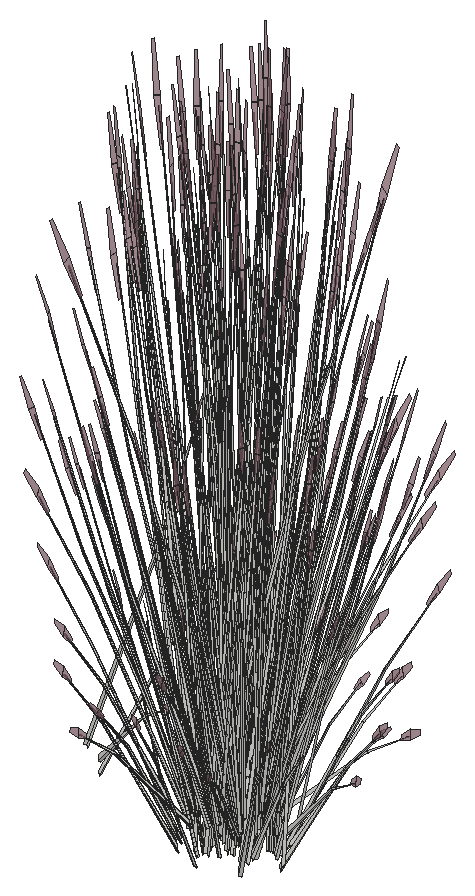
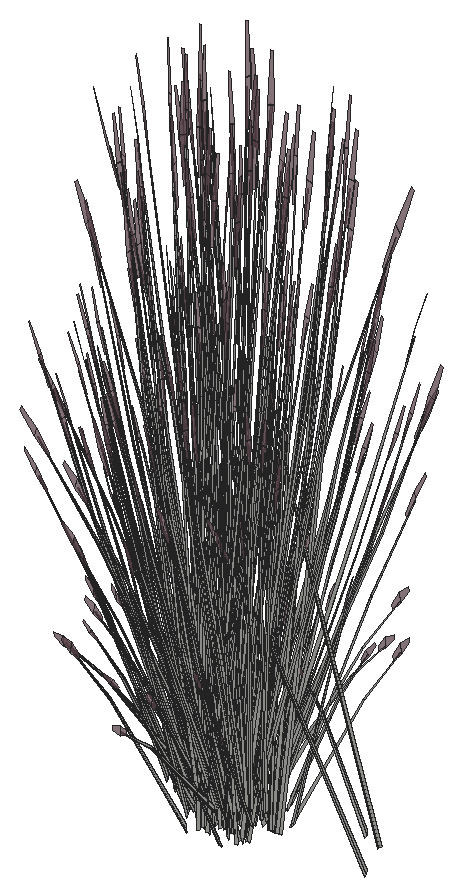
# SketchUp Ruby script. Lengths in inches.
U = 1.inch
M = Sketchup.active_model
def pt(a) = Geom::Point3d.new(a.map { |v| v * U })
def face(e, loops, mat)
  f = e.add_face(loops[0].map { |a| pt(a) })
  loops[1..].each { |l| e.add_face(l.map { |a| pt(a) }).erase! }
  f.material = f.back_material = mat if mat
  f
end
# faces: each face lists its corners as indices into pts; further lists are holes
def faces(e, pts, list, mat = nil) = list.each { |f| face(e, (f[0].is_a?(Array) ? f : [f]).map { |l| l.map { |i| pts[i] } }, mat) }
# xy, xz, yz: faces in a plane at the given z, y or x. An outline is a flat list of corners, or four numbers for a rectangle; further outlines are holes
def ring(l) = l.size == 4 ? [[l[0], l[1]], [l[2], l[1]], [l[2], l[3]], [l[0], l[3]]] : l.each_slice(2).to_a
def flat(e, list, mat, &to3) = list.each { |f| face(e, (f[0].is_a?(Array) ? f : [f]).map { |l| ring(l).map { |u, v| to3.(u, v) } }, mat) }
def xy(e, z, list, mat = nil) = flat(e, list, mat) { |x, y| [x, y, z] }
def xz(e, y, list, mat = nil) = flat(e, list, mat) { |x, z| [x, y, z] }
def yz(e, x, list, mat = nil) = flat(e, list, mat) { |y, z| [x, y, z] }
def lines(e, pts, list) = list.each { |a, b| e.add_line(pt(pts[a]), pt(pts[b])) }
# prism: a flat outline (further loops are holes) pulled along v
def prism(e, loops, v, mat = nil)
  f = face(e, loops, mat); d = Geom::Vector3d.new(v.map { |x| x * U })
  f.pushpull(f.normal.samedirection?(d) ? d.length : -d.length)
end
def box(e, o, s, mat = nil) = prism(e, [[o, [o[0] + s[0], o[1], o[2]], [o[0] + s[0], o[1] + s[1], o[2]], [o[0], o[1] + s[1], o[2]]]], [0, 0, s[2]], mat)
def at(x, y, z, deg = 0) = Geom::Transformation.translation(pt([x, y, z])) * Geom::Transformation.rotation(ORIGIN, Z_AXIS, deg.degrees)
def axes(o, x, y, z) = Geom::Transformation.new([*x, 0, *y, 0, *z, 0, *pt(o).to_a, 1])
def part(name) = M.definitions.add(name)
# library, detail: a bought-in or finely detailed component or shape, given as its bounding box
def library(name, o, s) = part(name).tap { |d| box(d.entities, o, s) }
def detail(e, o, s) = box(e.add_group.entities, o, s)
def put(e, d, t, mat = nil) = e.add_instance(d, t).tap { |i| i.material = mat if mat }
def group(e, t, mat = nil) = e.add_group.tap { |g| g.transformation = t; g.material = mat if mat }.entities
root = M.entities
M.materials.add("LightPink_Translucent").color = [144, 107, 117]
M.materials["LightPink_Translucent"].alpha = 0.75
c1 = part("blade")
p = [[2.15,0.21,22],[0,0.17,0],[0.09,0.45,0],[2.18,0.31,22],[2.29,0.31,22],[0.38,0.45,0],
  [2.48,0.24,33],[2.49,0.24,33],[2.48,0.22,33]]
faces(c1.entities,p,[[0,1,2,3],[4,5,2,3],[6,3,4,7],[8,0,3,6]])
c2 = part("seeds")
p = [[0.3,-0.1,1.38],[-0.01,-0.03,1.59],[-0.01,-0.03,0.03],[0.14,-0.07,-0.07],[0.29,-0.03,3],[0.15,0.01,3.11]]
faces(c2.entities,p,[[0,1,2,3],[1,0,4,5]],"LightPink_Translucent")
c3 = part("blade with seeds")
put(c3.entities,c1,at(0,0,0))
put(c3.entities,c2,axes([2.4,0.25,30.99],[1.5799,-0.05474,1.17369],[-0.12525,1.92788,0.29478],[-0.07173,-0.02425,1.56792]))
put(root,c3,axes([496.08,108.5625,4.17],[0.66765,-0.26986,-0.71045],[0.37208,0.55551,0.08574],[0.32259,-0.0631,1.00501]))
put(root,c3,axes([506.71,109.3125,3.875],[0.19519,0.55794,-0.51099],[-0.73919,0.0976,-0.3958],[-0.21183,0.14986,0.97773]))
put(root,c3,axes([506.92,106.35,3.92],[0.03826,-0.46465,0.0643],[0.57772,0.01274,0.50621],[-0.2213,-0.04862,0.77189]))
put(root,c3,axes([505.5625,110.32,3.91],[-0.01889,0.12092,1.74944],[0.53598,0.42065,-0.27667],[-0.14032,0.19892,0.14031]))
put(root,c3,axes([508.56,108.91,1.25],[-0.79037,-0.10018,-0.62353],[0.16679,-0.61794,-0.16365],[-0.23587,-0.07488,1.37633]))
put(root,c3,axes([508.7,105.54,4.62],[-0.50709,0.58578,-0.13619],[-0.73436,-0.33748,-0.75594],[-0.25527,-0.1655,1.14864]))
put(root,c3,axes([498.33,107.97,3.91],[0.10543,-0.09307,1.74944],[-0.13495,-0.57092,-0.27667],[0.26455,-0.10825,0.14031]))
put(root,c3,axes([507.31,106.69,4.24],[0.43232,0.38257,0.35414],[-0.49364,0.36215,-0.4572],[-0.25081,-0.0551,0.87481]))
put(root,c3,axes([508.48,106.02,4.17],[-0.64788,-0.29534,-0.71045],[0.46044,-0.51755,0.08574],[-0.23473,-0.17635,1.00501]))
put(root,c3,axes([508.18,106.03,3.875],[-0.74975,0.14525,-0.51099],[-0.13115,-0.55007,-0.3958],[-0.20138,-0.15763,0.97773]))
put(root,c3,axes([497.11,109.38,1.78],[-0.18299,-0.15028,1.43002],[0.23809,-0.49714,-0.30754],[0.37023,0.06735,0.61141]))
put(root,c3,axes([507.52,110.08,1.21],[-0.7111,-0.30552,-0.49651],[0.42504,-0.54784,0],[-0.16196,-0.06958,1.57504]))
put(root,c3,axes([507.21,105.53,0.6875],[-0.0736,0.08049,1.76342],[-0.74378,0.17355,-0.26939],[-0.17968,-0.15788,0.30037]))
put(root,c3,axes([506.37,108.91,4.23],[0.70283,0.33692,-0.1216],[-0.40491,0.48793,-0.67495],[-0.19857,0.16961,1.02557]))
put(root,c3,axes([507.95,110.45,1.57],[-0.47504,0.61229,0],[-0.79476,-0.34146,-0.51607],[-0.18101,-0.07777,1.63711]))
put(root,c3,axes([505.21,110.38,4.84],[0.67048,0.16311,-0.06488],[-0.20625,0.50201,-0.29416],[-0.10966,0.07622,0.97024]))
put(root,c3,axes([506.71,108.96,4.24],[0.66138,-0.08733,0.35414],[0.17464,0.49921,-0.4572],[-0.18953,0.13408,0.87481]))
put(root,c3,axes([507.09,111.34,1.78],[0.23977,-0.09639,1.43002],[0.59198,0.29065,-0.30754],[-0.1762,0.25149,0.61141]))
put(root,c3,axes([506.75,105.84,1.32],[-0.21918,0.49894,-0.03893],[-0.6746,-0.15348,-0.17649],[-0.10242,-0.08161,0.58215]))
put(root,c3,axes([508.5,104.15,3.9],[-0.01417,0.07324,1.77383],[-0.6991,0.2658,-0.16761],[-0.20573,-0.13587,0.31391]))
put(root,c3,axes([507.75,105.21,1.78],[-0.04601,0.19989,1.43002],[-0.67263,0.16733,-0.30754],[-0.15723,-0.25836,0.61141]))
put(root,c3,axes([507.97,105.73,3.07],[0.17368,0.19618,1.71376],[-0.80256,0.16516,0.13857],[-0.18139,-0.30799,0.73262]))
put(root,c3,axes([509.45,109,1.86],[-0.76714,0.40567,-0.29095],[-0.51013,-0.57321,-0.50002],[-0.18927,-0.05821,1.59708]))
put(root,c3,axes([507.33,110.29,3.93],[-0.54105,-0.41691,0.48003],[0.57458,-0.35956,0.3958],[-0.0998,0.1956,0.9933]))
put(root,c3,axes([508.26,105.63,3.72],[-0.11735,-0.49217,-0.35414],[0.67083,-0.12996,0.4572],[-0.18018,-0.14104,0.87481]))
put(root,c3,axes([506.38,108.12,1.57],[-0.95008,0,0],[0,-0.68292,-0.51607],[0,-0.15554,1.63711]))
put(root,c3,axes([507.72,109.85,1.22],[-0.17848,-0.53243,-0.30978],[0.70886,-0.15119,0.30978],[-0.1429,-0.0614,1.38974]))
put(root,c3,axes([507.14,110.25,3.92],[-0.62439,-0.02847,0.0643],[0.01712,-0.42991,0.50621],[-0.06534,0.16468,0.77189]))
put(root,c3,axes([507.33,110.41,3.72],[-0.5141,0.32171,-0.35414],[-0.48666,-0.36734,0.4572],[-0.07405,0.18664,0.87481]))
put(root,c3,axes([509.96,109.45,1.25],[-0.51177,0.45928,-0.62353],[-0.63575,-0.41646,-0.16365],[-0.20507,0.11457,1.37633]))
put(root,c3,axes([508.65,106.03,4.24],[0.11735,0.49217,0.35414],[-0.67083,0.12996,-0.4572],[-0.18018,-0.14104,0.87481]))
put(root,c3,axes([505.5,111.56,3.9],[0.0862,-0.03689,1.77383],[0.71245,0.24539,-0.16761],[-0.01674,0.20431,0.31391]))
put(root,c3,axes([507.12,107.94,1.52],[-0.70674,0.51372,0.30756],[-0.70717,-0.50832,-0.36492],[-0.02468,-0.14589,1.64885]))
put(root,c3,axes([510.03,109.36,2.52],[0.65659,0.2464,1.51261],[-0.64324,0.53082,0.59816],[-0.28812,-0.31461,1.26806]))
put(root,c3,axes([507.52,104.89,1.96],[0.39634,0.21267,1.1486],[-0.57721,0.12784,0.84392],[-0.1235,-0.16344,0.25299]))
put(root,c3,axes([510.32,109.1875,1.66],[-0.74193,-0.49181,-0.25192],[0.6243,-0.55226,0.5513],[-0.19979,0.05753,1.68216]))
put(root,c3,axes([508.97,108.72,1.4],[-0.45644,-0.51287,-0.44739],[0.69137,-0.36116,0.21531],[-0.14771,-0.06346,1.43643]))
put(root,c3,axes([507.68,110.07,4.53],[-0.01977,0.56521,-0.7886],[-0.83252,-0.03796,0.09517],[-0.08786,0.23945,1.11556]))
put(root,c3,axes([507.66,111.66,1.96],[-0.01966,-0.36332,1.1486],[0.49135,0.25914,0.84392],[-0.09663,0.17317,0.25299]))
put(root,c3,axes([508.35,105.45,4.29],[0.84639,-0.15705,0.53763],[0.14689,0.61608,0.4433],[-0.19906,-0.18157,1.11249]))
put(root,c3,axes([509.94,109.08,1.4],[-0.82508,0.03772,-0.44739],[-0.07462,-0.62614,0.21531],[-0.14771,0.06346,1.43643]))
put(root,c3,axes([508.55,105.58,3.92],[0.34533,-0.38816,0.0643],[0.49176,0.22599,0.50621],[-0.15898,-0.12445,0.77189]))
put(root,c3,axes([508.36,110.13,1.67],[0.7111,0.30552,0.49651],[-0.42504,0.54784,0],[-0.16196,-0.06958,1.57504]))
put(root,c3,axes([509.03,109.01,1.63],[0.20138,-0.72405,-0.23429],[0.95485,0.12621,0.51271],[-0.16685,-0.09999,1.5644]))
put(root,c3,axes([509.38,109.18,1.81],[-0.14658,0.54532,0.1448],[-0.71613,-0.09466,-0.41347],[-0.13033,-0.05599,1.26744]))
put(root,c3,axes([509.3,104.43,3.91],[-0.11621,-0.08567,1.74944],[-0.77555,0.05431,-0.27667],[-0.12378,-0.20491,0.14031]))
put(root,c3,axes([510.81,110.7,1.21],[-0.7111,0.30552,-0.49651],[-0.42504,-0.54784,0],[-0.16196,0.06958,1.57504]))
put(root,c3,axes([506.6,107.66,1.21],[0,-0.61104,-0.49651],[0.85008,0,0],[0,-0.13917,1.57504]))
put(root,c3,axes([506.96,108.22,1.67],[0,0.61104,0.49651],[-0.85008,0,0],[0,-0.13917,1.57504]))
put(root,c3,axes([510.85,110.54,1.39],[-0.46912,-0.61443,-0.05142],[0.79476,-0.34146,0.51607],[-0.19584,0.0585,1.6363]))
put(root,c3,axes([507.84,110.26,4.2],[0.54391,0.41056,-0.5672],[-0.57458,0.35956,-0.43934],[-0.08276,0.2086,1.08528]))
put(root,c3,axes([510.64,110.46,1.22],[-0.70886,-0.15119,-0.30978],[0.17848,-0.53243,0.30978],[-0.1429,0.0614,1.38974]))
put(root,c3,axes([507.6,109.95,4.24],[0.5141,-0.32171,0.35414],[0.48666,0.36734,-0.4572],[-0.07405,0.18664,0.87481]))
put(root,c3,axes([508.82,108.36,1.86],[-0.85568,-0.29155,-0.29095],[0.41201,-0.61537,-0.50002],[-0.02689,-0.15109,1.59708]))
put(root,c3,axes([511.05,108.18,2.03],[-0.02076,-0.57531,1.41272],[0.93937,0.14913,0.59816],[-0.22217,0.31481,1.3335]))
put(root,c3,axes([507.27,110.04,4.59],[0.83505,0.03027,-0.13498],[-0.02282,0.57322,-0.74919],[-0.05801,0.22077,1.13838]))
put(root,c3,axes([507.25,110.875,2.02],[0.69024,-0.1082,0.06507],[0.15868,0.43593,-0.86304],[-0.04376,0.22067,0.7736]))
put(root,c3,axes([510.52,108.92,1.86],[0.08854,0.69723,-0.29095],[-0.92215,0.04216,-0.50002],[-0.16238,0.09287,1.59708]))
put(root,c3,axes([508.4375,107.74,1.29],[-0.31203,-0.62659,-0.69835],[0.89884,-0.22566,-0.18329],[-0.03449,-0.21218,1.54149]))
put(root,c3,axes([510.48,105.75,4.23],[-0.74352,0.28449,-0.1216],[-0.36538,-0.50492,-0.67495],[-0.0981,-0.21277,1.02557]))
put(root,c3,axes([509.84,105.78,3.875],[-0.7469,-0.15318,-0.51099],[0.25601,-0.52518,-0.3958],[-0.06849,-0.21144,0.97773]))
put(root,c3,axes([508.46,109.67,3.07],[-0.0186,-0.23452,1.71376],[0.80601,0.15558,0.13857],[-0.04985,0.33422,0.73262]))
put(root,c3,axes([506.96,107.67,1.22],[0.53038,-0.38124,-0.30978],[0.53038,0.38124,0.30978],[0,-0.1228,1.38974]))
put(root,c3,axes([509.36,105.2,1.32],[-0.52505,0.35054,-0.03893],[-0.48109,-0.38392,-0.17649],[-0.03387,-0.10878,0.58215]))
put(root,c3,axes([509.15,108.66,1.55],[0.96033,0.12874,0.45755],[-0.19544,0.7271,0.17955],[-0.14034,-0.07021,1.58856]))
put(root,c3,axes([508.9,108.53,1.91],[-0.36864,0.55059,0.44739],[-0.76598,-0.26498,-0.21531],[0,-0.12692,1.43643]))
put(root,c3,axes([510.11,105.88,4.17],[-0.36264,-0.49684,-0.71045],[0.74649,-0.27689,0.08574],[-0.0848,-0.24006,1.00501]))
put(root,c3,axes([508.63,109.82,1.67],[0.81646,-0.16218,0.17642],[0.20161,0.60355,0.35086],[-0.07282,-0.08794,1.60407]))
put(root,c3,axes([509.68,109.92,1.39],[-0.76598,-0.27433,0],[0.36864,-0.57001,0],[0,0,1.62707]))
put(root,c3,axes([510.26,105.95,4.24],[-0.22906,0.4699,0.35414],[-0.66828,-0.13705,-0.4572],[-0.06128,-0.18919,0.87481]))
put(root,c3,axes([511.45,110.61,1.57],[0.47504,0.61229,0],[-0.79476,0.34146,-0.51607],[-0.18101,0.07777,1.63711]))
put(root,c3,axes([509.03,110.87,4.26],[-0.74868,-0.15974,0.53283],[0.25601,-0.52518,0.43934],[0.04499,0.20653,1.10256]))
put(root,c3,axes([508.84,110.91,3.92],[-0.55987,0.20767,0.0643],[-0.27403,-0.37869,0.50621],[0.05407,0.16693,0.77189]))
put(root,c3,axes([511.06,109.86,1.67],[0.21949,-0.60727,0.17642],[0.8032,0.17185,0.35086],[-0.13875,0.00296,1.60407]))
put(root,c3,axes([510.6875,109.05,1.81],[0.56134,0.36712,0.1448],[-0.46823,0.41419,-0.41347],[-0.13033,0.05599,1.26744]))
put(root,c3,axes([510.49,108.6,1.49],[-0.70674,-0.52593,-0.06131],[0.70717,-0.52625,0],[-0.02468,-0.01837,1.75571]))
put(root,c3,axes([510.67,108.78,1.91],[0.82508,-0.03772,0.44739],[0.07462,0.62614,-0.21531],[-0.14771,0.06346,1.43643]))
put(root,c3,axes([510.875,110.22,1.52],[0.95122,0.19861,0.30756],[-0.23797,0.7099,-0.36492],[-0.15744,0.08885,1.64885]))
put(root,c3,axes([509.49,104.78,0.6875],[-0.12744,0.02202,1.76342],[-0.70477,-0.24781,-0.26939],[0.01183,-0.2067,0.30037]))
put(root,c3,axes([511.29,110.18,1.67],[0.7111,-0.30552,0.49651],[0.42504,0.54784,0],[-0.16196,0.06958,1.57504]))
put(root,c3,axes([510.18,105.46,3.72],[0.22906,-0.4699,-0.35414],[0.66828,0.13705,0.4572],[-0.06128,-0.18919,0.87481]))
put(root,c3,axes([509.0625,107.99,1.55],[0.33034,0.68327,0.45755],[-0.94388,0.2376,0.17955],[0.01154,-0.12555,1.58856]))
put(root,c3,axes([508.91,107.91,1.4],[0.36864,-0.55059,-0.44739],[0.76598,0.26498,0.21531],[0,-0.12692,1.43643]))
put(root,c3,axes([509.86,109.68,1.4],[-0.24791,-0.5268,0],[0.70791,-0.18448,0],[0,0,1.54371]))
put(root,c3,axes([508.95,110.79,0.6875],[0.12297,-0.03325,1.76342],[0.73967,0.18301,-0.26939],[0.02163,0.20626,0.30037]))
put(root,c3,axes([509.12,110.98,3.72],[-0.22906,0.4699,-0.35414],[-0.66828,-0.13705,0.4572],[0.06128,0.18919,0.87481]))
put(root,c3,axes([510.86,108.64,1.4],[-0.36864,0.55059,-0.44739],[-0.76598,-0.26498,0.21531],[0,0.12692,1.43643]))
put(root,c3,axes([510.46,105.52,3.92],[0.55987,-0.20767,0.0643],[0.27403,0.37869,0.50621],[-0.05407,-0.16693,0.77189]))
put(root,c3,axes([508.64,111.8125,3.91],[0.09631,0.0984,1.74944],[0.77725,0.03866,-0.27667],[0.07816,0.217,0.14031]))
put(root,c3,axes([512.3125,108.31,1.67],[-0.59697,-0.44509,0.17642],[0.60159,-0.4317,0.35086],[-0.06593,0.0909,1.60407]))
put(root,c3,axes([510.25,108.05,1.4],[0,-0.70701,0],[0.95008,0,0],[0,0,1.79456]))
put(root,c3,axes([510.26,105.56,3.93],[0.74868,0.15974,0.48003],[-0.25601,0.52518,0.3958],[-0.04499,-0.20653,0.9933]))
put(root,c3,axes([509.37,108.18,1.625],[0.8561,0.29616,0.24065],[-0.41201,0.61537,0.50002],[0,-0.14185,1.60543]))
put(root,c3,axes([510.73,108.33,1.48],[0,0.70667,-0.05637],[-0.95008,0,0],[0,0.02221,1.79368]))
put(root,c3,axes([509.09,107.77,1.91],[-0.82508,0.03772,0.44739],[-0.07462,-0.62614,-0.21531],[0.14771,-0.06346,1.43643]))
put(root,c3,axes([509.04,110.48,4.24],[0.22906,-0.4699,0.35414],[0.66828,0.13705,-0.4572],[0.06128,0.18919,0.87481]))
put(root,c3,axes([508.71,106.69,1.67],[-0.21949,0.60727,0.17642],[-0.8032,-0.17185,0.35086],[0.13875,-0.00296,1.60407]))
put(root,c3,axes([510.27,109.7,1.48],[0.33034,0.70197,-0.06012],[-0.94388,0.24598,0],[0.01154,0.02451,1.72173]))
put(root,c3,axes([508.3125,105.94,1.57],[-0.47504,-0.61229,0],[0.79476,-0.34146,-0.51607],[0.18101,-0.07777,1.63711]))
put(root,c3,axes([509.1875,110.56,4.17],[0.36264,0.49684,-0.71045],[-0.74649,0.27689,0.08574],[0.0848,0.24006,1.00501]))
put(root,c3,axes([513,108.78,1.39],[-0.94962,-0.00489,-0.04976],[0,-0.68292,0.49943],[-0.02984,0.15546,1.58352]))
put(root,c3,axes([511.14,106.72,1.67],[-0.81646,0.16218,0.17642],[-0.20161,-0.60355,0.35086],[0.07282,0.08794,1.60407]))
put(root,c3,axes([510.3,104.46,1.96],[0.09747,0.35631,1.1486],[-0.54071,-0.19735,0.84392],[0.05818,-0.18244,0.25299]))
put(root,c3,axes([509.94,112.16,4.84],[0.52505,-0.35054,-0.06488],[0.48109,0.38392,-0.29416],[0.03387,0.10878,0.97024]))
put(root,c3,axes([509.8,107.6,1.55],[-0.62999,0.55453,0.45755],[-0.74845,-0.4895,0.17955],[0.15188,-0.05534,1.58856]))
put(root,c3,axes([510.875,108.48,1.41],[0.53038,0.39469,0],[-0.53038,0.39469,0],[0,0,1.69266]))
put(root,c3,axes([510.87,108.02,1.91],[0.36864,-0.55059,0.44739],[0.76598,0.26498,-0.21531],[0,0.12692,1.43643]))
put(root,c3,axes([510.55,109.93,1.4],[0.76598,0.27433,0],[-0.36864,0.57001,0],[0,0,1.74954]))
put(root,c3,axes([509.46,110.66,3.875],[0.7469,0.15318,-0.51099],[-0.25601,0.52518,-0.3958],[0.06849,0.21144,0.97773]))
put(root,c3,axes([508.82,110.68,4.23],[0.74352,-0.28449,-0.1216],[0.36538,0.50492,-0.67495],[0.0981,0.21277,1.02557]))
put(root,c3,axes([510.62,107.89,1.57],[-0.96033,-0.12874,0.49198],[0.19544,-0.7271,0.19306],[0.14034,0.07021,1.70813]))
put(root,c3,axes([512.62,105.04,3.9],[-0.07716,0.04667,1.77383],[-0.75601,-0.15746,-0.16761],[-0.02737,-0.20368,0.31391]))
put(root,c3,axes([512.02,106.39,4.23],[-0.83505,-0.03027,-0.1216],[0.02282,-0.57322,-0.67495],[0.05801,-0.22077,1.02557]))
put(root,c3,axes([512.8,108.88,1.22],[-0.53038,0.38124,-0.30978],[-0.53038,-0.38124,0.30978],[0,0.1228,1.38974]))
put(root,c3,axes([511.29,108.81,1.29],[0.2786,0.55945,-0.69212],[-0.80253,0.20149,-0.18165],[0.03079,0.18945,1.52773]))
put(root,c3,axes([510.9,108.21,1.4],[0.85008,0,0],[0,0.63259,0],[0,0,1.78407]))
put(root,c3,axes([511.7,106.48,4.24],[-0.5141,0.32171,0.35414],[-0.48666,-0.36734,-0.4572],[0.07405,-0.18664,0.87481]))
put(root,c3,axes([510.08,107.51,1.91],[-0.45644,-0.51287,0.44739],[0.69137,-0.36116,-0.21531],[0.14771,0.06346,1.43643]))
put(root,c3,axes([509.25,107.63,1.86],[-0.08854,-0.69723,-0.29095],[0.92215,-0.04216,-0.50002],[0.16238,-0.09287,1.59708]))
put(root,c3,axes([511.19,108.14,1.81],[0.70791,-0.1782,0.1448],[0.24791,0.50885,-0.41347],[0,0.11199,1.26744]))
put(root,c3,axes([511.45,106.18,3.875],[-0.54391,-0.41056,-0.51099],[0.57458,-0.35956,-0.3958],[0.08276,-0.2086,0.97773]))
put(root,c3,axes([510.95,108.18,1.86],[0.85568,0.29155,-0.29095],[-0.41201,0.61537,-0.50002],[0.02689,0.15109,1.59708]))
put(root,c3,axes([509.125,106.09,1.22],[0.70886,0.15119,-0.30978],[-0.17848,0.53243,0.30978],[0.1429,-0.0614,1.38974]))
put(root,c3,axes([511.1,105.45,1.78],[-0.21597,0.12368,1.43002],[-0.64681,-0.21647,-0.30754],[0.1199,-0.26922,0.61141]))
put(root,c3,axes([512.8,108.32,1.67],[0,-0.61104,0.49651],[0.85008,0,0],[0,0.13917,1.57504]))
put(root,c3,axes([513.17,108.89,1.21],[0,0.61104,-0.49651],[-0.85008,0,0],[0,0.13917,1.57504]))
put(root,c3,axes([510.9,110.74,3.93],[-0.75571,0.14023,0.48003],[-0.13115,-0.55007,0.3958],[0.17773,0.16212,0.9933]))
put(root,c3,axes([508.96,105.85,1.21],[0.7111,-0.30552,-0.49651],[0.42504,0.54784,0],[0.16196,-0.06958,1.57504]))
put(root,c3,axes([510.75,110.85,3.92],[-0.34533,0.38816,0.0643],[-0.49176,-0.22599,0.50621],[0.15898,0.12445,0.77189]))
put(root,c3,axes([509.88,109.57,3.07],[-0.17368,-0.19618,1.71376],[0.80256,-0.16516,0.13857],[0.18139,0.30799,0.73262]))
put(root,c3,axes([510.38,107.37,1.81],[0.14658,-0.54532,0.1448],[0.71613,0.09466,-0.41347],[0.13033,0.05599,1.26744]))
put(root,c3,axes([511.4,106.42,1.67],[-0.7111,-0.30552,0.49651],[0.42504,-0.54784,0],[0.16196,0.06958,1.57504]))
put(root,c3,axes([511.625,106.36,4.17],[0.01977,-0.56521,-0.71045],[0.83252,0.03796,0.08574],[0.08786,-0.23945,1.00501]))
put(root,c3,axes([510.78,109.61,1.38],[0.79769,-0.20732,-0.19198],[0.2803,0.59721,0.00008],[0.08805,-0.02292,1.73897]))
put(root,c3,axes([510.65,110.41,4.24],[-0.11735,-0.49217,0.35414],[0.67083,-0.12996,-0.4572],[0.18018,0.14104,0.87481]))
put(root,c3,axes([510.8,107.83,1.4],[0.45644,0.51287,-0.44739],[-0.69137,0.36116,0.21531],[0.14771,0.06346,1.43643]))
put(root,c3,axes([511.1,107.57,3.67],[-0.65655,-0.31748,1.38283],[0.69326,-0.49431,0.59665],[0.21183,0.29789,1.33663]))
put(root,c3,axes([511.97,106.02,3.72],[0.5141,-0.32171,-0.35414],[0.48666,0.36734,0.4572],[0.07405,-0.18664,0.87481]))
put(root,c3,axes([509.99,111.09,3.9],[0.00225,-0.07398,1.77383],[0.65113,-0.32638,-0.16761],[0.22617,0.1165,0.31391]))
put(root,c3,axes([512.16,106.1875,3.92],[0.62439,0.02847,0.0643],[-0.01712,0.42991,0.50621],[0.06534,-0.16468,0.77189]))
put(root,c3,axes([512.09,110.16,1.96],[-0.4278,-0.1757,1.1486],[0.5524,-0.17852,0.84392],[0.14899,0.15122,0.25299]))
put(root,c3,axes([510.57,109.97,1.78],[0.01341,-0.20255,1.43002],[0.64074,-0.22625,-0.30754],[0.1978,0.24243,0.61141]))
put(root,c3,axes([512.78,105.48,3.91],[-0.00733,-0.12161,1.74944],[-0.61946,-0.35147,-0.27667],[0.09577,-0.21306,0.14031]))
put(root,c3,axes([509.8,107.1,1.25],[0.51177,-0.45928,-0.62353],[0.63575,0.41646,-0.16365],[0.20507,-0.11457,1.37633]))
put(root,c3,axes([511.96,106.15,3.93],[0.54105,0.41691,0.48003],[-0.57458,0.35956,0.3958],[0.0998,-0.1956,0.9933]))
put(root,c3,axes([512.05,106.69,1.22],[0.17848,0.53243,-0.30978],[-0.70886,0.15119,0.30978],[0.1429,0.0614,1.38974]))
put(root,c3,axes([513.38,108.43,1.57],[0.95008,0,0],[0,0.68292,-0.51607],[0,0.15554,1.63711]))
put(root,c3,axes([510.3125,107.54,1.86],[0.76714,-0.40567,-0.29095],[0.51013,0.57321,-0.50002],[0.18927,0.05821,1.59708]))
put(root,c3,axes([512.16,110.96,1.86],[-0.48723,-0.01916,1.0506],[0.32177,-0.40701,0.58006],[0.19248,0.1446,0.8241]))
put(root,c3,axes([512.59,107.47,4.24],[-0.66138,0.08733,0.35414],[-0.17464,-0.49921,-0.4572],[0.18953,-0.13408,0.87481]))
put(root,c3,axes([510.6875,106.08,3.07],[-0.14147,0.21002,1.71376],[-0.59349,-0.43464,0.13857],[0.26773,-0.27089,0.73262]))
put(root,c3,axes([510.59,110.66,4.23],[0.45276,-0.52302,-0.1216],[0.65568,0.30132,-0.67495],[0.22792,0.14777,1.02557]))
put(root,c3,axes([508.375,107.18,0.79],[-0.74787,0.24464,1.28929],[-0.23804,-0.70192,0.50096],[0.45924,0.01168,1.46642]))
put(root,c3,axes([512.93,107.52,4.23],[-0.70283,-0.33692,-0.1216],[0.40491,-0.48793,-0.67495],[0.19857,-0.16961,1.02557]))
put(root,c3,axes([511.12,110.4,3.875],[0.74975,-0.14525,-0.51099],[0.13115,0.55007,-0.3958],[0.20138,0.15763,0.97773]))
put(root,c3,axes([511.8125,106.1,1.57],[0.47504,-0.61229,0],[0.79476,0.34146,-0.51607],[0.18101,0.07777,1.63711]))
put(root,c3,axes([512.61,105.83,0.6875],[-0.11372,-0.04814,1.76342],[-0.29211,-0.53779,-0.26939],[0.19706,-0.14594,0.30037]))
put(root,c3,axes([511.98,109.74,4.24],[-0.43232,-0.38257,0.35414],[0.49364,-0.36215,-0.4572],[0.25081,0.0551,0.87481]))
put(root,c3,axes([512.24,106.47,1.21],[0.7111,0.30552,-0.49651],[-0.42504,0.54784,0],[0.16196,0.06958,1.57504]))
put(root,c3,axes([512.375,110.09,3.92],[-0.03826,0.46465,0.0643],[-0.57772,-0.01274,0.50621],[0.2213,0.04862,0.77189]))
put(root,c3,axes([512.21,110.8125,0.6875],[0.05536,-0.08822,1.76342],[0.69692,-0.25981,-0.26939],[0.21129,0.13447,0.30037]))
put(root,c3,axes([512.43,109.94,3.93],[-0.56024,0.40262,0.48003],[-0.48318,-0.42758,0.3958],[0.26285,0.07427,0.9933]))
put(root,c3,axes([512.58,107.12,3.875],[-0.19519,-0.55794,-0.51099],[0.73919,-0.0976,-0.3958],[0.21183,-0.14986,0.97773]))
put(root,c3,axes([513.88,110,3.12],[-0.14542,-0.51365,-0.03492],[0.68734,-0.11809,-0.15832],[0.14353,0.03256,0.52218]))
put(root,c3,axes([512.7,108.67,4.24],[-0.63144,-0.17046,0.35414],[0.18417,-0.49731,-0.4572],[0.25423,-0.0456,0.87481]))
put(root,c3,axes([511.21,107.64,1.25],[0.79037,0.10018,-0.62353],[-0.16679,0.61794,-0.16365],[0.23587,0.07488,1.37633]))
put(root,c3,axes([514.57,108,1.45],[-0.47106,-0.39072,-0.06488],[0.51591,-0.35801,-0.29416],[0.14618,-0.02521,0.97024]))
put(root,c3,axes([513.49,106.01,1.96],[-0.25308,0.31105,1.1486],[-0.21753,-0.4179,0.84392],[0.20902,-0.10472,0.25299]))
put(root,c3,axes([513.19,107.4,3.92],[0.52161,0.25698,0.0643],[-0.30368,0.36595,0.50621],[0.16723,-0.11831,0.77189]))
put(root,c3,axes([513.04,107.29,3.93],[0.18844,0.56237,0.48003],[-0.73919,0.0976,0.3958],[0.21785,-0.13226,0.9933]))
put(root,c3,axes([511.04,108.96,3.07],[-0.28223,-0.10528,1.71376],[0.58406,-0.44165,0.13857],[0.36402,0.19924,0.73262]))
put(root,c3,axes([514.66,107.375,3.9],[-0.09924,-0.00464,1.77383],[-0.4121,-0.49725,-0.16761],[0.1655,-0.1635,0.31391]))
put(root,c3,axes([513.13,107.18,3.72],[0.66138,-0.08733,-0.35414],[0.17464,0.49921,0.4572],[0.18953,-0.13408,0.87481]))
put(root,c3,axes([512.6,107.35,4.17],[0.39688,-0.48213,-0.71045],[0.69548,0.34264,0.08574],[0.23697,-0.17468,1.00501]))
put(root,c3,axes([513.27,108.82,3.92],[0.27906,0.41663,0.0643],[-0.50888,0.20393,0.50621],[0.22432,-0.04024,0.77189]))
put(root,c3,axes([512.6,109.94,3.72],[0.43232,0.38257,-0.35414],[-0.49364,0.36215,0.4572],[0.25081,0.0551,0.87481]))
put(root,c3,axes([512.1,109.98,4.23],[0.04068,-0.62141,-0.1216],[0.77029,0.01698,-0.67495],[0.29667,0.04317,1.02557]))
put(root,c3,axes([512.96,108.84,4.23],[-0.38229,-0.5533,-0.1216],[0.6785,-0.2719,-0.67495],[0.28593,-0.073,1.02557]))
put(root,c3,axes([513.21,108.67,3.93],[-0.21466,0.55714,0.48003],[-0.70573,-0.19051,0.3958],[0.27753,-0.03348,0.9933]))
put(root,c3,axes([512.77,109.61,3.91],[0.16299,-0.01033,1.74944],[0.44707,-0.47471,-0.27667],[0.28992,0.06266,0.14031]))
put(root,c3,axes([512.93,108.36,3.875],[0.20584,-0.55581,-0.51099],[0.70573,0.19051,-0.3958],[0.28414,-0.05097,0.97773]))
put(root,c3,axes([514.7,108.71,1.96],[-0.46945,0.10088,1.1486],[0.22097,-0.4169,0.84392],[0.24904,0.02853,0.25299]))
put(root,c3,axes([513.18,106.9,1.78],[-0.27143,-0.0181,1.43002],[-0.27808,-0.48551,-0.30754],[0.33346,-0.13735,0.61141]))
put(root,c3,axes([513.36,108.61,3.72],[0.63144,0.17046,-0.35414],[-0.18417,0.49731,0.4572],[0.25423,-0.0456,0.87481]))
put(root,c3,axes([512.14,109.6875,4.17],[0.75952,0.01471,-0.71045],[-0.05101,0.61953,0.08574],[0.32177,0.06538,1.00501]))
put(root,c3,axes([513.68,108.52,1.17],[-0.48937,0.07333,1.41583],[-0.07789,-0.58369,0.08104],[0.34275,-0.08835,0.80566]))
put(root,c3,axes([514.22,108.13,0.6875],[-0.03971,-0.09277,1.76342],[0.27541,-0.54264,-0.26939],[0.27782,-0.00781,0.30037]))
put(root,c3,axes([514.48,110.48,3.9],[-0.0687,-0.05349,1.77383],[0.15029,-0.57341,-0.16761],[0.27062,-0.03664,0.31391]))
put(root,c3,axes([511.64,108,3.07],[-0.31515,0.01384,1.71376],[0.20907,-0.5998,0.13857],[0.44912,0.0371,0.73262]))
put(root,c3,axes([512.79,108.5625,4.17],[0.66765,-0.26986,-0.71045],[0.37208,0.55551,0.08574],[0.32259,-0.0631,1.00501]))
put(root,c3,axes([515.04,107.97,3.91],[0.10543,-0.09307,1.74944],[-0.13495,-0.57092,-0.27667],[0.26455,-0.10825,0.14031]))
put(root,c3,axes([513.82,109.38,1.78],[-0.18299,-0.15028,1.43002],[0.23809,-0.49714,-0.30754],[0.37023,0.06735,0.61141]))
